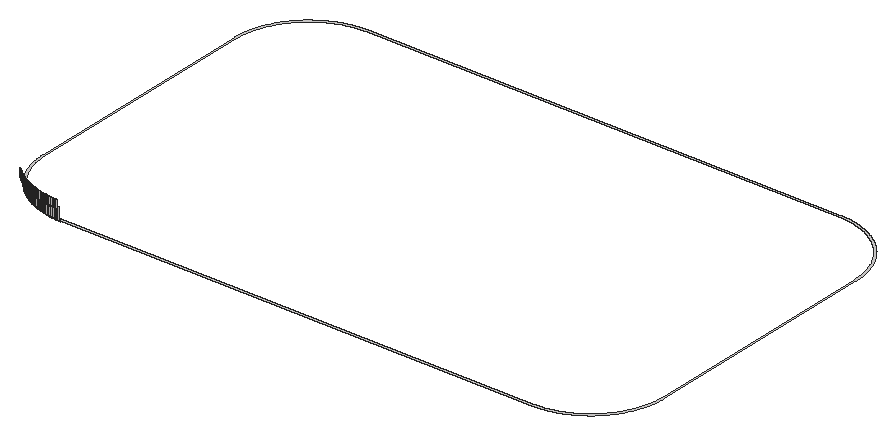
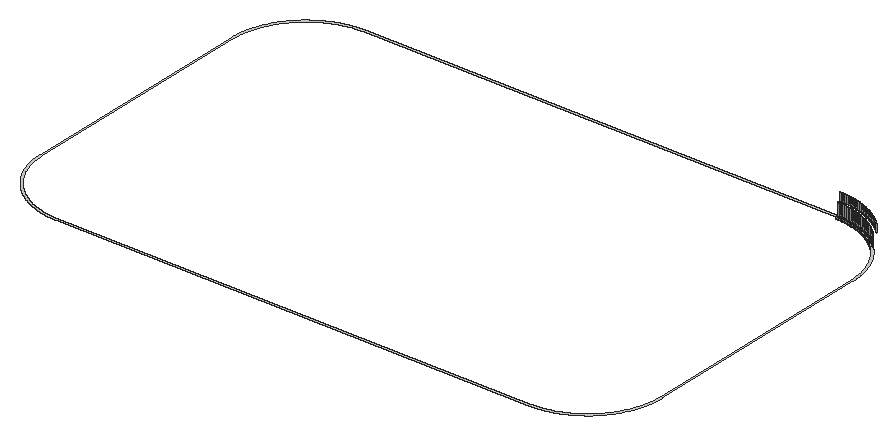
# SketchUp Ruby script. Lengths in inches.
U = 1.inch
M = Sketchup.active_model
def pt(a) = Geom::Point3d.new(a.map { |v| v * U })
def face(e, loops, mat)
  f = e.add_face(loops[0].map { |a| pt(a) })
  loops[1..].each { |l| e.add_face(l.map { |a| pt(a) }).erase! }
  f.material = f.back_material = mat if mat
  f
end
# faces: each face lists its corners as indices into pts; further lists are holes
def faces(e, pts, list, mat = nil) = list.each { |f| face(e, (f[0].is_a?(Array) ? f : [f]).map { |l| l.map { |i| pts[i] } }, mat) }
# xy, xz, yz: faces in a plane at the given z, y or x. An outline is a flat list of corners, or four numbers for a rectangle; further outlines are holes
def ring(l) = l.size == 4 ? [[l[0], l[1]], [l[2], l[1]], [l[2], l[3]], [l[0], l[3]]] : l.each_slice(2).to_a
def flat(e, list, mat, &to3) = list.each { |f| face(e, (f[0].is_a?(Array) ? f : [f]).map { |l| ring(l).map { |u, v| to3.(u, v) } }, mat) }
def xy(e, z, list, mat = nil) = flat(e, list, mat) { |x, y| [x, y, z] }
def xz(e, y, list, mat = nil) = flat(e, list, mat) { |x, z| [x, y, z] }
def yz(e, x, list, mat = nil) = flat(e, list, mat) { |y, z| [x, y, z] }
def lines(e, pts, list) = list.each { |a, b| e.add_line(pt(pts[a]), pt(pts[b])) }
# prism: a flat outline (further loops are holes) pulled along v
def prism(e, loops, v, mat = nil)
  f = face(e, loops, mat); d = Geom::Vector3d.new(v.map { |x| x * U })
  f.pushpull(f.normal.samedirection?(d) ? d.length : -d.length)
end
def box(e, o, s, mat = nil) = prism(e, [[o, [o[0] + s[0], o[1], o[2]], [o[0] + s[0], o[1] + s[1], o[2]], [o[0], o[1] + s[1], o[2]]]], [0, 0, s[2]], mat)
def at(x, y, z, deg = 0) = Geom::Transformation.translation(pt([x, y, z])) * Geom::Transformation.rotation(ORIGIN, Z_AXIS, deg.degrees)
def axes(o, x, y, z) = Geom::Transformation.new([*x, 0, *y, 0, *z, 0, *pt(o).to_a, 1])
def part(name) = M.definitions.add(name)
# library, detail: a bought-in or finely detailed component or shape, given as its bounding box
def library(name, o, s) = part(name).tap { |d| box(d.entities, o, s) }
def detail(e, o, s) = box(e.add_group.entities, o, s)
def put(e, d, t, mat = nil) = e.add_instance(d, t).tap { |i| i.material = mat if mat }
def group(e, t, mat = nil) = e.add_group.tap { |g| g.transformation = t; g.material = mat if mat }.entities
root = M.entities
M.materials.add("[Quartz Light Brown]").color = [215, 212, 212]
xy(root,487,[[[224.5,282.7,224.01,282.71,223.01,282.75,222.51,282.78,222.02,282.82,221.52,282.86,221.03,282.91,220.53,282.96,220.04,283.03,219.55,283.09,219.06,283.17,218.56,283.25,218.08,283.34,217.59,283.43,217.1,283.53,216.61,283.64,216.13,283.75,215.65,283.87,215.16,284,214.69,284.13,213.73,284.41,213.26,284.5625,212.79,284.72,212.32,284.88,211.38,285.22,210.92,285.41,210.46,285.59,209.54,285.99,209.09,286.19,208.64,286.4,208.19,286.62,207.75,286.84,207.31,287.07,206.43,287.55,206,287.79,205.57,288.04,205.15,288.3,204.72,288.5625,204.3,288.83,203.89,289.11,203.48,289.38,202.66,289.96,202.26,290.25,201.87,290.55,201.47,290.86,201.09,291.17,200.7,291.49,199.94,292.13,199.57,292.46,199.21,292.8,198.84,293.14,198.48,293.48,197.78,294.18,197.4375,294.54,197.1,294.91,196.76,295.27,196.43,295.65,196.1,296.02,195.78,296.4,194.85,297.57,194.55,297.96,194.26,298.37,193.97,298.77,193.68,299.18,193.4,299.59,193.13,300,192.86,300.42,192.6,300.85,192.34,301.27,192.09,301.7,191.85,302.13,191.6,302.57,191.14,303.45,190.92,303.89,190.7,304.34,190.49,304.79,190.29,305.25,190.09,305.7,189.89,306.16,189.71,306.62,189.52,307.08,189.18,308.02,188.86,308.96,188.71,309.43,188.56,309.91,188.43,310.39,188.29,310.87,188.05,311.83,187.9375,312.31,187.83,312.8,187.73,313.29,187.55,314.27,187.39,315.25,187.33,315.74,187.26,316.23,187.21,316.73,187.16,317.22,187.08,318.22,187.05,318.71,187.01,319.71,187,320.2,187,441.2,187.01,441.7,187.03,442.19,187.05,442.69,187.08,443.1875,187.12,443.68,187.16,444.18,187.21,444.67,187.26,445.17,187.33,445.66,187.39,446.15,187.47,446.65,187.55,447.14,187.73,448.11,187.83,448.6,187.9375,449.09,188.05,449.57,188.17,450.05,188.29,450.54,188.43,451.02,188.56,451.49,188.71,451.97,188.86,452.44,189.02,452.92,189.18,453.39,189.35,453.85,189.52,454.32,189.71,454.78,189.89,455.24,190.29,456.16,190.49,456.61,190.7,457.06,190.92,457.51,191.14,457.95,191.6,458.83,191.85,459.27,192.09,459.7,192.34,460.13,192.6,460.56,192.86,460.98,193.13,461.4,193.4,461.8125,193.68,462.22,194.26,463.04,194.55,463.4375,194.85,463.83,195.16,464.23,195.47,464.62,195.78,465,196.1,465.38,196.43,465.76,196.76,466.13,197.1,466.5,197.4375,466.86,197.78,467.22,198.48,467.92,198.84,468.27,199.21,468.61,199.57,468.94,199.94,469.27,200.32,469.6,200.7,469.92,201.09,470.23,201.47,470.54,201.87,470.85,202.26,471.15,202.66,471.44,203.48,472.02,203.89,472.3,204.3,472.57,204.72,472.84,205.15,473.1,205.57,473.36,206.43,473.86,206.87,474.1,207.75,474.56,208.19,474.78,208.64,475,209.54,475.42,210,475.62,210.92,476,211.38,476.18,212.32,476.52,213.26,476.84,213.73,476.99,214.21,477.14,214.69,477.27,215.16,477.41,215.65,477.53,216.13,477.65,216.61,477.76,217.1,477.87,217.59,477.97,218.08,478.06,218.56,478.15,219.06,478.23,219.55,478.31,220.04,478.375,220.53,478.4375,221.03,478.49,221.52,478.54,222.02,478.58,222.51,478.62,223.01,478.65,223.51,478.67,224.01,478.6875,224.5,478.7,464.5,478.7,464.99,478.6875,465.49,478.67,465.99,478.65,466.49,478.62,466.98,478.58,467.48,478.54,467.97,478.49,468.47,478.4375,468.96,478.375,469.45,478.31,469.94,478.23,470.44,478.15,470.92,478.06,471.41,477.97,471.9,477.87,472.39,477.76,472.87,477.65,473.35,477.53,473.84,477.41,474.31,477.27,474.79,477.14,475.27,476.99,475.74,476.84,476.68,476.52,477.62,476.18,478.08,476,479,475.62,479.46,475.42,480.36,475,480.81,474.78,481.25,474.56,482.13,474.1,482.57,473.86,483.43,473.36,483.85,473.1,484.28,472.84,484.7,472.57,485.11,472.3,485.52,472.02,486.34,471.44,486.74,471.15,487.13,470.85,487.53,470.54,487.91,470.23,488.3,469.92,488.68,469.6,489.06,469.27,489.43,468.94,489.79,468.61,490.16,468.27,490.52,467.92,491.22,467.22,491.5625,466.86,491.9,466.5,492.24,466.13,492.57,465.76,492.9,465.38,493.22,465,493.53,464.62,493.84,464.23,494.15,463.83,494.45,463.4375,494.74,463.04,495.32,462.22,495.6,461.8125,495.87,461.4,496.14,460.98,496.4,460.56,496.66,460.13,496.91,459.7,497.15,459.27,497.4,458.83,497.86,457.95,498.08,457.51,498.3,457.06,498.51,456.61,498.71,456.16,499.11,455.24,499.29,454.78,499.48,454.32,499.65,453.85,499.82,453.39,499.98,452.92,500.14,452.44,500.29,451.97,500.44,451.49,500.57,451.02,500.71,450.54,500.83,450.05,500.95,449.57,501.0625,449.09,501.17,448.6,501.27,448.11,501.45,447.14,501.53,446.65,501.61,446.15,501.67,445.66,501.74,445.17,501.79,444.67,501.84,444.18,501.88,443.68,501.92,443.1875,501.95,442.69,501.97,442.19,501.99,441.7,502,441.2,502,320.2,501.99,319.71,501.95,318.71,501.92,318.22,501.84,317.22,501.79,316.73,501.74,316.23,501.67,315.74,501.61,315.25,501.45,314.27,501.27,313.29,501.17,312.8,501.0625,312.31,500.95,311.83,500.71,310.87,500.57,310.39,500.44,309.91,500.29,309.43,500.14,308.96,499.82,308.02,499.48,307.08,499.29,306.62,499.11,306.16,498.91,305.7,498.71,305.25,498.51,304.79,498.3,304.34,498.08,303.89,497.86,303.45,497.4,302.57,497.15,302.13,496.91,301.7,496.66,301.27,496.4,300.85,496.14,300.42,495.87,300,495.6,299.59,495.32,299.18,495.03,298.77,494.74,298.37,494.45,297.96,494.15,297.57,493.22,296.4,492.9,296.02,492.57,295.65,492.24,295.27,491.9,294.91,491.5625,294.54,491.22,294.18,490.52,293.48,490.16,293.14,489.79,292.8,489.43,292.46,489.06,292.13,488.3,291.49,487.91,291.17,487.53,290.86,487.13,290.55,486.74,290.25,486.34,289.96,485.52,289.38,485.11,289.11,484.7,288.83,484.28,288.5625,483.85,288.3,483.43,288.04,483,287.79,482.57,287.55,481.69,287.07,481.25,286.84,480.81,286.62,480.36,286.4,479.91,286.19,479.46,285.99,478.54,285.59,478.08,285.41,477.62,285.22,476.68,284.88,476.21,284.72,475.74,284.5625,475.27,284.41,474.31,284.13,473.84,284,473.35,283.87,472.87,283.75,472.39,283.64,471.9,283.53,471.41,283.43,470.92,283.34,470.44,283.25,469.94,283.17,469.45,283.09,468.96,283.03,468.47,282.96,467.97,282.91,467.48,282.86,466.98,282.82,466.49,282.78,465.99,282.75,464.99,282.71,464.5,282.7],[224.52,283.7,464.48,283.7,464.97,283.71,465.45,283.73,465.9375,283.75,466.42,283.78,466.9,283.82,467.39,283.86,467.87,283.9,469.31,284.08,470.27,284.24,470.74,284.32,471.22,284.41,471.69,284.51,472.17,284.61,472.64,284.72,473.58,284.96,474.04,285.09,474.51,285.22,474.97,285.37,475.43,285.51,475.89,285.66,476.35,285.82,476.81,285.99,477.26,286.16,478.16,286.52,478.61,286.71,479.05,286.9,479.49,287.1,479.93,287.31,480.36,287.52,480.8,287.73,481.23,287.96,481.65,288.18,482.08,288.42,482.92,288.9,483.33,289.15,484.15,289.67,484.56,289.9375,484.96,290.21,485.35,290.49,485.75,290.77,486.14,291.05,486.52,291.35,486.91,291.64,487.28,291.95,487.66,292.25,488.03,292.57,488.4,292.88,488.76,293.2,489.12,293.53,489.47,293.86,489.82,294.2,490.5,294.88,490.84,295.23,491.17,295.59,491.5,295.94,491.82,296.31,492.14,296.67,492.45,297.04,492.75,297.42,493.06,297.79,493.35,298.18,493.65,298.5625,493.93,298.95,494.22,299.35,494.49,299.74,494.76,300.14,495.03,300.55,495.55,301.37,495.8,301.78,496.28,302.62,496.52,303.05,496.74,303.47,496.97,303.9,497.18,304.34,497.4,304.77,497.8,305.65,498,306.1,498.18,306.54,498.37,306.99,498.71,307.89,498.88,308.35,499.04,308.81,499.1875,309.27,499.34,309.73,499.48,310.19,499.61,310.66,499.74,311.125,499.86,311.59,499.98,312.0625,500.09,312.54,500.29,313.48,500.47,314.44,500.54,314.91,500.62,315.39,500.8,316.83,500.84,317.32,500.89,317.8,500.95,318.76,500.97,319.25,500.99,319.73,501,320.22,501,441.19,500.99,441.67,500.97,442.15,500.95,442.64,500.89,443.6,500.84,444.09,500.8,444.57,500.62,446.01,500.54,446.49,500.47,446.97,500.38,447.44,500.29,447.92,500.19,448.39,500.09,448.87,499.98,449.34,499.74,450.28,499.61,450.74,499.48,451.21,499.34,451.67,499.1875,452.13,499.04,452.59,498.88,453.05,498.71,453.51,498.37,454.41,498.18,454.86,498,455.31,497.4,456.63,497.18,457.07,496.97,457.5,496.74,457.93,496.52,458.36,495.8,459.62,495.55,460.03,495.03,460.85,494.76,461.26,494.22,462.06,493.93,462.45,493.65,462.84,493.35,463.23,493.06,463.61,492.75,463.99,492.45,464.36,492.14,464.73,491.82,465.1,491.5,465.46,491.17,465.82,490.84,466.17,490.5,466.52,489.82,467.2,489.47,467.54,489.12,467.87,488.76,468.2,488.4,468.52,488.03,468.84,487.66,469.15,487.28,469.46,486.91,469.76,486.52,470.06,486.14,470.35,485.75,470.63,485.35,470.92,484.96,471.19,484.56,471.47,483.33,472.25,482.92,472.5,482.08,472.98,481.65,473.22,481.23,473.45,480.8,473.67,480.36,473.89,479.93,474.1,478.61,474.7,478.16,474.88,477.71,475.07,476.81,475.41,476.35,475.58,475.89,475.74,474.97,476.04,474.51,476.18,474.04,476.3125,473.58,476.44,473.11,476.5625,472.64,476.68,472.17,476.79,471.69,476.89,471.22,476.99,470.74,477.08,470.27,477.17,469.79,477.25,469.31,477.32,467.87,477.5,467.39,477.55,466.9,477.59,466.42,477.62,465.9375,477.65,465.45,477.67,464.97,477.6875,464.48,477.7,224.52,477.7,224.03,477.6875,223.55,477.67,223.0625,477.65,222.58,477.62,222.1,477.59,221.61,477.55,221.13,477.5,219.69,477.32,219.21,477.25,218.73,477.17,218.26,477.08,217.78,476.99,217.31,476.89,216.83,476.79,216.36,476.68,215.89,476.5625,215.42,476.44,214.96,476.3125,214.49,476.18,214.03,476.04,213.11,475.74,212.65,475.58,212.19,475.41,211.29,475.07,210.84,474.88,210.39,474.7,209.07,474.1,208.64,473.89,208.2,473.67,207.77,473.45,207.35,473.22,206.92,472.98,206.08,472.5,205.67,472.25,204.44,471.47,204.04,471.19,203.65,470.92,203.25,470.63,202.86,470.35,202.48,470.06,202.09,469.76,201.72,469.46,201.34,469.15,200.97,468.84,200.6,468.52,200.24,468.2,199.88,467.87,199.53,467.54,199.18,467.2,198.5,466.52,198.16,466.17,197.83,465.82,197.5,465.46,197.18,465.1,196.86,464.73,196.55,464.36,196.25,463.99,195.94,463.61,195.65,463.23,195.35,462.84,195.07,462.45,194.78,462.06,194.24,461.26,193.97,460.85,193.45,460.03,193.2,459.62,192.48,458.36,192.26,457.93,192.03,457.5,191.82,457.07,191.6,456.63,191,455.31,190.82,454.86,190.63,454.41,190.29,453.51,190.12,453.05,189.96,452.59,189.8125,452.13,189.66,451.67,189.52,451.21,189.39,450.74,189.26,450.28,189.02,449.34,188.91,448.87,188.81,448.39,188.71,447.92,188.62,447.44,188.53,446.97,188.46,446.49,188.38,446.01,188.2,444.57,188.16,444.09,188.11,443.6,188.05,442.64,188.03,442.15,188.01,441.67,188,441.19,188,320.22,188.01,319.73,188.03,319.25,188.05,318.76,188.11,317.8,188.16,317.32,188.2,316.83,188.38,315.39,188.46,314.91,188.53,314.44,188.71,313.48,188.91,312.54,189.02,312.0625,189.14,311.59,189.26,311.125,189.39,310.66,189.52,310.19,189.66,309.73,189.8125,309.27,189.96,308.81,190.12,308.35,190.29,307.89,190.63,306.99,190.82,306.54,191,306.1,191.2,305.65,191.6,304.77,191.82,304.34,192.03,303.9,192.26,303.47,192.48,303.05,192.72,302.62,193.2,301.78,193.45,301.37,193.97,300.55,194.24,300.14,194.51,299.74,194.78,299.35,195.07,298.95,195.35,298.5625,195.65,298.18,195.94,297.79,196.25,297.42,196.55,297.04,196.86,296.67,197.18,296.31,197.5,295.94,197.83,295.59,198.16,295.23,198.5,294.88,199.18,294.2,199.53,293.86,199.88,293.53,200.24,293.2,200.6,292.88,200.97,292.57,201.34,292.25,201.72,291.95,202.09,291.64,202.48,291.35,202.86,291.05,203.25,290.77,203.65,290.49,204.04,290.21,204.44,289.9375,204.85,289.67,205.67,289.15,206.08,288.9,206.92,288.42,207.35,288.18,207.77,287.96,208.2,287.73,208.64,287.52,209.07,287.31,209.51,287.1,209.95,286.9,210.39,286.71,210.84,286.52,211.74,286.16,212.19,285.99,212.65,285.82,213.11,285.66,213.57,285.51,214.03,285.37,214.49,285.22,214.96,285.09,215.42,284.96,216.36,284.72,216.83,284.61,217.31,284.51,217.78,284.41,218.26,284.32,218.73,284.24,219.69,284.08,221.13,283.9,221.61,283.86,222.1,283.82,222.58,283.78,223.0625,283.75,223.55,283.73,224.03,283.71]]],"[Quartz Light Brown]")
xz(root,281.2,[[224.48,493,225,497]],"[Quartz Light Brown]")
xz(root,282.7,[[224.5,487,225,493]],"[Quartz Light Brown]")
xz(root,283.7,[[224.52,486,225,487]],"[Quartz Light Brown]")
p = [[223.0625,283.75,486],[223.55,283.73,486],[223.55,283.73,487],[223.0625,283.75,487],[224.03,283.71,486],[224.03,283.71,487],
  [224.52,283.7,486],[224.52,283.7,487],[221.61,283.86,486],[222.1,283.82,486],[222.1,283.82,487],[221.61,283.86,487],
  [222.58,283.78,486],[222.58,283.78,487],[220.65,283.96,486],[221.13,283.9,486],[221.13,283.9,487],[220.65,283.96,487],
  [219.69,284.08,486],[220.17,284.02,486],[220.17,284.02,487],[219.69,284.08,487],[219.21,284.16,486],[219.21,284.16,487],
  [218.26,284.32,486],[218.73,284.24,486],[218.73,284.24,487],[218.26,284.32,487],[217.78,284.41,486],[217.78,284.41,487],
  [217.31,284.51,486],[217.31,284.51,487],[216.83,284.61,486],[216.83,284.61,487],[216.36,284.72,486],[216.36,284.72,487],
  [215.89,284.84,486],[215.89,284.84,487],[215.42,284.96,486],[215.42,284.96,487],[214.96,285.09,486],[214.96,285.09,487],
  [214.49,285.22,486],[214.49,285.22,487],[214.03,285.37,486],[214.03,285.37,487],[213.57,285.51,486],[213.57,285.51,487],
  [213.11,285.66,486],[213.11,285.66,487],[212.65,285.82,486],[212.65,285.82,487],[212.19,285.99,486],[212.19,285.99,487],
  [211.74,286.16,486],[211.74,286.16,487],[211.29,286.34,486],[211.29,286.34,487],[210.84,286.52,486],[210.84,286.52,487],
  [210.39,286.71,486],[210.39,286.71,487],[209.95,286.9,486],[209.95,286.9,487],[209.51,287.1,486],[209.51,287.1,487],
  [209.07,287.31,486],[209.07,287.31,487],[208.64,287.52,486],[208.64,287.52,487],[208.2,287.73,486],[208.2,287.73,487],
  [207.77,287.96,486],[207.77,287.96,487],[207.35,288.18,486],[207.35,288.18,487],[206.92,288.42,486],[206.92,288.42,487],
  [206.5,288.66,486],[206.5,288.66,487],[206.08,288.9,486],[206.08,288.9,487],[205.67,289.15,486],[205.67,289.15,487],
  [205.26,289.41,486],[205.26,289.41,487],[204.85,289.67,486],[204.85,289.67,487],[204.44,289.9375,486],[204.44,289.9375,487],
  [204.04,290.21,486],[204.04,290.21,487],[203.65,290.49,486],[203.65,290.49,487],[203.25,290.77,486],[203.25,290.77,487],
  [202.86,291.05,486],[202.86,291.05,487],[202.48,291.35,486],[202.48,291.35,487],[202.09,291.64,486],[202.09,291.64,487],
  [201.72,291.95,486],[201.72,291.95,487],[201.34,292.25,486],[201.34,292.25,487],[200.97,292.57,486],[200.97,292.57,487],
  [200.6,292.88,486],[200.6,292.88,487],[200.24,293.2,486],[200.24,293.2,487],[199.88,293.53,486],[199.88,293.53,487],
  [199.53,293.86,486],[199.53,293.86,487],[199.18,294.2,486],[199.18,294.2,487],[198.84,294.54,486],[198.84,294.54,487],
  [198.5,294.88,486],[198.5,294.88,487],[198.16,295.23,486],[198.16,295.23,487],[197.83,295.59,486],[197.83,295.59,487],
  [223.51,282.73,487],[223.51,282.73,493],[223.01,282.75,493],[223.01,282.75,487],[224.01,282.71,487],[224.01,282.71,493],
  [224.5,282.7,487],[224.5,282.7,493],[222.02,282.82,487],[222.02,282.82,493],[221.52,282.86,493],[221.52,282.86,487],
  [222.51,282.78,487],[222.51,282.78,493],[221.03,282.91,487],[221.03,282.91,493],[220.53,282.96,493],[220.53,282.96,487],
  [220.04,283.03,487],[220.04,283.03,493],[219.55,283.09,493],[219.55,283.09,487],[219.06,283.17,493],[219.06,283.17,487],
  [218.56,283.25,487],[218.56,283.25,493],[218.08,283.34,493],[218.08,283.34,487],[217.59,283.43,493],[217.59,283.43,487],
  [217.1,283.53,493],[217.1,283.53,487],[216.61,283.64,493],[216.61,283.64,487],[216.13,283.75,493],[216.13,283.75,487],
  [215.65,283.87,493],[215.65,283.87,487],[215.16,284,493],[215.16,284,487],[214.69,284.13,493],[214.69,284.13,487],
  [214.21,284.27,493],[214.21,284.27,487],[213.73,284.41,493],[213.73,284.41,487],[213.26,284.5625,493],[213.26,284.5625,487],
  [212.79,284.72,493],[212.79,284.72,487],[212.32,284.88,493],[212.32,284.88,487],[211.85,285.05,493],[211.85,285.05,487],
  [211.38,285.22,493],[211.38,285.22,487],[210.92,285.41,493],[210.92,285.41,487],[210.46,285.59,493],[210.46,285.59,487],
  [210,285.79,493],[210,285.79,487],[209.54,285.99,493],[209.54,285.99,487],[209.09,286.19,493],[209.09,286.19,487],
  [208.64,286.4,493],[208.64,286.4,487],[208.19,286.62,493],[208.19,286.62,487],[207.75,286.84,493],[207.75,286.84,487],
  [207.31,287.07,493],[207.31,287.07,487],[206.87,287.31,493],[206.87,287.31,487],[206.43,287.55,493],[206.43,287.55,487],
  [206,287.79,493],[206,287.79,487],[205.57,288.04,493],[205.57,288.04,487],[205.15,288.3,493],[205.15,288.3,487],
  [204.72,288.5625,493],[204.72,288.5625,487],[204.3,288.83,493],[204.3,288.83,487],[203.89,289.11,493],[203.89,289.11,487],
  [203.48,289.38,493],[203.48,289.38,487],[203.07,289.67,493],[203.07,289.67,487],[202.66,289.96,493],[202.66,289.96,487],
  [202.26,290.25,493],[202.26,290.25,487],[201.87,290.55,493],[201.87,290.55,487],[201.47,290.86,493],[201.47,290.86,487],
  [201.09,291.17,493],[201.09,291.17,487],[200.7,291.49,493],[200.7,291.49,487],[200.32,291.81,493],[200.32,291.81,487],
  [199.94,292.13,493],[199.94,292.13,487],[199.57,292.46,493],[199.57,292.46,487],[199.21,292.8,493],[199.21,292.8,487],
  [198.84,293.14,493],[198.84,293.14,487],[198.48,293.48,493],[198.48,293.48,487],[198.13,293.83,493],[198.13,293.83,487],
  [222.93,281.26,493],[223.45,281.23,493],[223.45,281.23,497],[222.93,281.26,497],[223.97,281.21,493],[223.97,281.21,497],
  [224.48,281.2,493],[224.48,281.2,497],[221.39,281.37,493],[221.9,281.32,493],[221.9,281.32,497],[221.39,281.37,497],
  [222.42,281.29,493],[222.42,281.29,497],[220.36,281.47,493],[220.87,281.42,493],[220.87,281.42,497],[220.36,281.47,497],
  [219.33,281.61,493],[219.84,281.54,493],[219.84,281.54,497],[219.33,281.61,497],[218.82,281.6875,493],[218.82,281.6875,497],
  [218.3125,281.77,493],[218.3125,281.77,497],[217.8,281.86,493],[217.8,281.86,497],[217.29,281.96,493],[217.29,281.96,497],
  [216.79,282.0625,493],[216.79,282.0625,497],[216.28,282.17,493],[216.28,282.17,497],[215.78,282.29,493],[215.78,282.29,497],
  [215.28,282.42,493],[215.28,282.42,497],[214.78,282.55,493],[214.78,282.55,497],[214.28,282.68,493],[214.28,282.68,497],
  [213.78,282.83,493],[213.78,282.83,497],[213.29,282.98,493],[213.29,282.98,497],[212.79,283.13,493],[212.79,283.13,497],
  [212.3,283.3,493],[212.3,283.3,497],[211.81,283.47,493],[211.81,283.47,497],[211.33,283.64,493],[211.33,283.64,497],
  [210.84,283.82,493],[210.84,283.82,497],[210.36,284.01,493],[210.36,284.01,497],[209.88,284.21,493],[209.88,284.21,497],
  [209.41,284.41,493],[209.41,284.41,497],[208.93,284.62,493],[208.93,284.62,497],[208.46,284.83,493],[208.46,284.83,497],
  [207.99,285.05,493],[207.99,285.05,497],[207.53,285.27,493],[207.53,285.27,497],[207.07,285.51,493],[207.07,285.51,497],
  [206.61,285.74,493],[206.61,285.74,497],[206.15,285.99,493],[206.15,285.99,497],[205.7,286.24,493],[205.7,286.24,497],
  [205.25,286.49,493],[205.25,286.49,497],[204.8,286.75,493],[204.8,286.75,497],[204.36,287.02,493],[204.36,287.02,497],
  [203.92,287.29,493],[203.92,287.29,497],[203.49,287.57,493],[203.49,287.57,497],[203.05,287.86,493],[203.05,287.86,497],
  [202.625,288.15,493],[202.625,288.15,497],[202.2,288.44,493],[202.2,288.44,497],[201.78,288.74,493],[201.78,288.74,497],
  [201.37,289.05,493],[201.37,289.05,497],[200.95,289.36,493],[200.95,289.36,497],[200.55,289.68,493],[200.55,289.68,497],
  [200.14,290,493],[200.14,290,497],[199.74,290.33,493],[199.74,290.33,497],[199.35,290.66,493],[199.35,290.66,497],
  [198.96,291,493],[198.96,291,497],[198.57,291.35,493],[198.57,291.35,497],[198.1875,291.7,493],[198.1875,291.7,497],
  [197.81,292.05,493],[197.81,292.05,497],[225,282.7,493],[225,282.7,495]]
faces(root,p,[[0,1,2,3],[1,4,5,2],[4,6,7,5],[8,9,10,11],[9,12,13,10],[12,0,3,13],[14,15,16,17],[15,8,11,16],
  [18,19,20,21],[19,14,17,20],[22,18,21,23],[24,25,26,27],[25,22,23,26],[28,24,27,29],[30,28,29,31],[32,30,31,33],
  [34,32,33,35],[36,34,35,37],[38,36,37,39],[40,38,39,41],[42,40,41,43],[44,42,43,45],[46,44,45,47],[48,46,47,49],
  [50,48,49,51],[52,50,51,53],[54,52,53,55],[56,54,55,57],[58,56,57,59],[60,58,59,61],[62,60,61,63],[64,62,63,65],
  [66,64,65,67],[68,66,67,69],[70,68,69,71],[72,70,71,73],[74,72,73,75],[76,74,75,77],[78,76,77,79],[80,78,79,81],
  [82,80,81,83],[84,82,83,85],[86,84,85,87],[88,86,87,89],[90,88,89,91],[92,90,91,93],[94,92,93,95],[96,94,95,97],
  [98,96,97,99],[100,98,99,101],[102,100,101,103],[104,102,103,105],[106,104,105,107],[108,106,107,109],[110,108,109,111],[112,110,111,113],
  [114,112,113,115],[116,114,115,117],[118,116,117,119],[120,118,119,121],[122,120,121,123],[124,122,123,125],[126,127,128,129],[130,131,127,126],
  [132,133,131,130],[134,135,136,137],[138,139,135,134],[129,128,139,138],[140,141,142,143],[137,136,141,140],[144,145,146,147],[143,142,145,144],
  [147,146,148,149],[150,151,152,153],[149,148,151,150],[153,152,154,155],[155,154,156,157],[157,156,158,159],[159,158,160,161],[161,160,162,163],
  [163,162,164,165],[165,164,166,167],[167,166,168,169],[169,168,170,171],[171,170,172,173],[173,172,174,175],[175,174,176,177],[177,176,178,179],
  [179,178,180,181],[181,180,182,183],[183,182,184,185],[185,184,186,187],[187,186,188,189],[189,188,190,191],[191,190,192,193],[193,192,194,195],
  [195,194,196,197],[197,196,198,199],[199,198,200,201],[201,200,202,203],[203,202,204,205],[205,204,206,207],[207,206,208,209],[209,208,210,211],
  [211,210,212,213],[213,212,214,215],[215,214,216,217],[217,216,218,219],[219,218,220,221],[221,220,222,223],[223,222,224,225],[225,224,226,227],
  [227,226,228,229],[229,228,230,231],[231,230,232,233],[233,232,234,235],[235,234,236,237],[237,236,238,239],[239,238,240,241],[241,240,242,243],
  [243,242,244,245],[246,247,248,249],[247,250,251,248],[250,252,253,251],[254,255,256,257],[255,258,259,256],[258,246,249,259],[260,261,262,263],
  [261,254,257,262],[264,265,266,267],[265,260,263,266],[268,264,267,269],[270,268,269,271],[272,270,271,273],[274,272,273,275],[276,274,275,277],
  [278,276,277,279],[280,278,279,281],[282,280,281,283],[284,282,283,285],[286,284,285,287],[288,286,287,289],[290,288,289,291],[292,290,291,293],
  [294,292,293,295],[296,294,295,297],[298,296,297,299],[300,298,299,301],[302,300,301,303],[304,302,303,305],[306,304,305,307],[308,306,307,309],
  [310,308,309,311],[312,310,311,313],[314,312,313,315],[316,314,315,317],[318,316,317,319],[320,318,319,321],[322,320,321,323],[324,322,323,325],
  [326,324,325,327],[328,326,327,329],[330,328,329,331],[332,330,331,333],[334,332,333,335],[336,334,335,337],[338,336,337,339],[340,338,339,341],
  [342,340,341,343],[344,342,343,345],[346,344,345,347],[348,346,347,349],[350,348,349,351],[352,350,351,353],[354,352,353,355],[356,354,355,357],
  [358,356,357,359],[360,358,359,361]],"[Quartz Light Brown]")
lines(root,p,[[362,363]])
